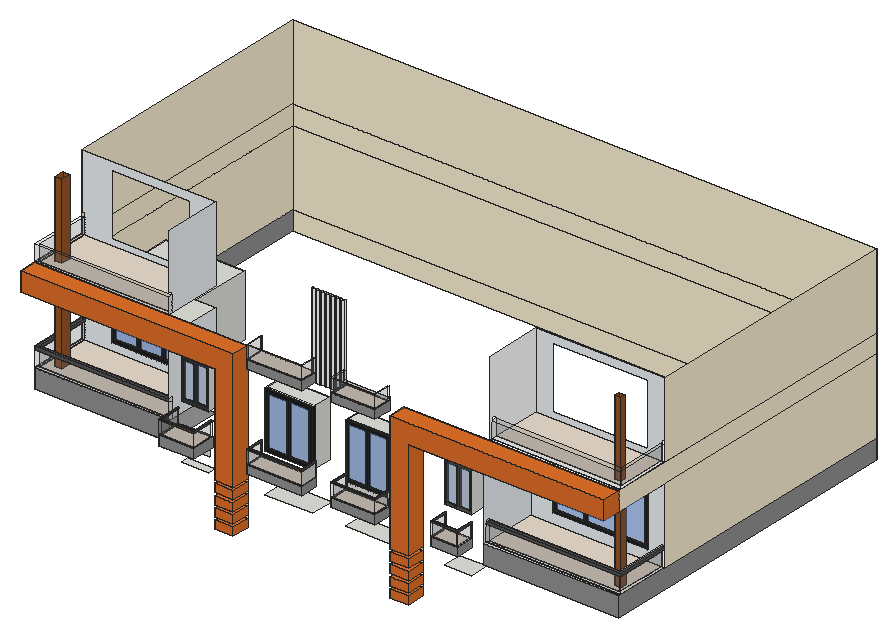
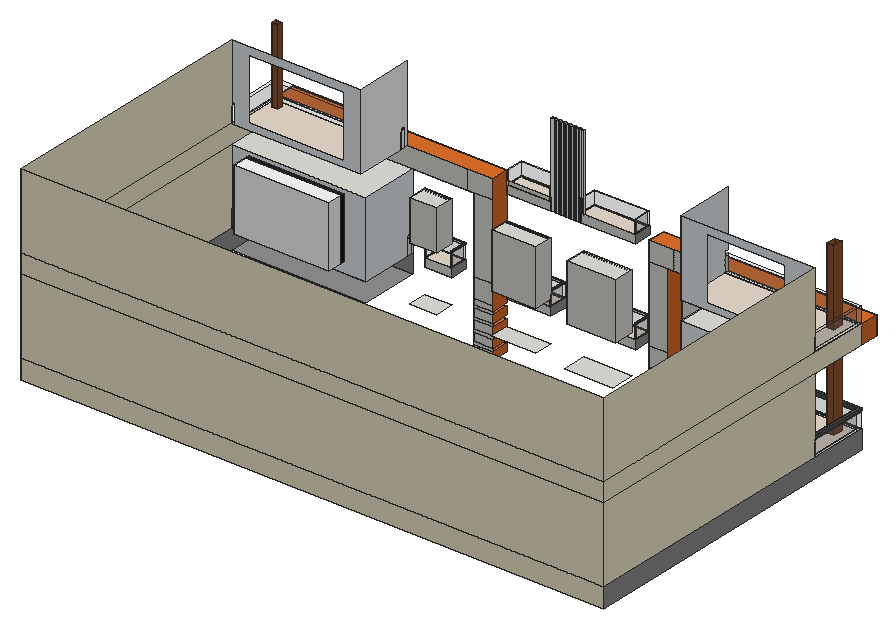
# SketchUp Ruby script. Lengths in inches.
U = 1.inch
M = Sketchup.active_model
def pt(a) = Geom::Point3d.new(a.map { |v| v * U })
def face(e, loops, mat)
  f = e.add_face(loops[0].map { |a| pt(a) })
  loops[1..].each { |l| e.add_face(l.map { |a| pt(a) }).erase! }
  f.material = f.back_material = mat if mat
  f
end
# faces: each face lists its corners as indices into pts; further lists are holes
def faces(e, pts, list, mat = nil) = list.each { |f| face(e, (f[0].is_a?(Array) ? f : [f]).map { |l| l.map { |i| pts[i] } }, mat) }
# xy, xz, yz: faces in a plane at the given z, y or x. An outline is a flat list of corners, or four numbers for a rectangle; further outlines are holes
def ring(l) = l.size == 4 ? [[l[0], l[1]], [l[2], l[1]], [l[2], l[3]], [l[0], l[3]]] : l.each_slice(2).to_a
def flat(e, list, mat, &to3) = list.each { |f| face(e, (f[0].is_a?(Array) ? f : [f]).map { |l| ring(l).map { |u, v| to3.(u, v) } }, mat) }
def xy(e, z, list, mat = nil) = flat(e, list, mat) { |x, y| [x, y, z] }
def xz(e, y, list, mat = nil) = flat(e, list, mat) { |x, z| [x, y, z] }
def yz(e, x, list, mat = nil) = flat(e, list, mat) { |y, z| [x, y, z] }
def lines(e, pts, list) = list.each { |a, b| e.add_line(pt(pts[a]), pt(pts[b])) }
# prism: a flat outline (further loops are holes) pulled along v
def prism(e, loops, v, mat = nil)
  f = face(e, loops, mat); d = Geom::Vector3d.new(v.map { |x| x * U })
  f.pushpull(f.normal.samedirection?(d) ? d.length : -d.length)
end
def box(e, o, s, mat = nil) = prism(e, [[o, [o[0] + s[0], o[1], o[2]], [o[0] + s[0], o[1] + s[1], o[2]], [o[0], o[1] + s[1], o[2]]]], [0, 0, s[2]], mat)
def at(x, y, z, deg = 0) = Geom::Transformation.translation(pt([x, y, z])) * Geom::Transformation.rotation(ORIGIN, Z_AXIS, deg.degrees)
def axes(o, x, y, z) = Geom::Transformation.new([*x, 0, *y, 0, *z, 0, *pt(o).to_a, 1])
def part(name) = M.definitions.add(name)
# library, detail: a bought-in or finely detailed component or shape, given as its bounding box
def library(name, o, s) = part(name).tap { |d| box(d.entities, o, s) }
def detail(e, o, s) = box(e.add_group.entities, o, s)
def put(e, d, t, mat = nil) = e.add_instance(d, t).tap { |i| i.material = mat if mat }
def group(e, t, mat = nil) = e.add_group.tap { |g| g.transformation = t; g.material = mat if mat }.entities
root = M.entities
M.materials.add("Generic").color = [146, 146, 146]
M.materials.add("Generic\#3").color = [226, 112, 41]
M.materials.add("Generic\#4").color = [237, 241, 244]
M.materials.add("Generic\#5").color = [249, 239, 211]
M.materials.add("Generic\#7").color = [232, 220, 205]
M.materials.add("[Color M00]").color = [255, 255, 255]
M.materials.add("[Color M06]").color = [86, 86, 86]
M.materials.add("[Color M07]").color = [58, 58, 58]
M.materials.add("[Color M08]").color = [30, 30, 30]
M.materials.add("[Translucent Glass Blue]").color = [98, 147, 234]
M.materials["[Translucent Glass Blue]"].alpha = 0.27
M.materials.add("[Translucent Glass Blue]1").color = [100, 149, 237]
M.materials["[Translucent Glass Blue]1"].alpha = 0.5
M.materials.add("[Translucent Glass Gray]").color = [119, 119, 119]
M.materials["[Translucent Glass Gray]"].alpha = 0.16
M.materials.add("[Wood Cherry Original]").color = [150, 85, 41]
M.materials.add("[Wood Cherry Original]1").color = [152, 86, 42]
c1 = part("Group\#11")
xy(c1.entities,0,[[0,0,175.8125,6]],"[Color M08]")
xy(c1.entities,7.33,[[7.33,0,56.16,3],[63.49,0,112.32,3],[119.65,0,168.48,3]],"[Color M08]")
xy(c1.entities,131.1,[[7.33,0,56.16,3],[63.49,0,112.32,3],[119.65,0,168.48,3]],"[Color M08]")
xy(c1.entities,138.4375,[[0,0,175.8125,6]],"[Color M08]")
xz(c1.entities,0,[[[0,0,175.8125,0,175.8125,131.1,168.48,131.1,168.48,7.33,119.65,7.33,119.65,131.1,175.8125,131.1,175.8125,138.4375,0,138.4375],[7.33,7.33,56.16,131.1],[63.49,7.33,112.32,131.1]]],"[Color M08]")
xz(c1.entities,3,[[7.33,7.33,56.16,131.1],[63.49,7.33,112.32,131.1],[119.65,7.33,168.48,131.1]],"[Translucent Glass Blue]1")
xz(c1.entities,6,[[0,0,175.8125,138.4375]])
yz(c1.entities,0,[[0,0,6,138.4375]],"[Color M08]")
yz(c1.entities,7.33,[[0,7.33,3,131.1]],"[Color M08]")
yz(c1.entities,56.16,[[0,7.33,3,131.1]],"[Color M08]")
yz(c1.entities,63.49,[[0,7.33,3,131.1]],"[Color M08]")
yz(c1.entities,112.32,[[0,7.33,3,131.1]],"[Color M08]")
yz(c1.entities,119.65,[[0,7.33,3,131.1]],"[Color M08]")
yz(c1.entities,168.48,[[0,7.33,3,131.1]],"[Color M08]")
yz(c1.entities,175.8125,[[0,0,6,138.4375]],"[Color M08]")
c2 = part("Group\#10")
xy(c2.entities,0,[[0,0,98.1875,6]],"[Color M08]")
xy(c2.entities,5.79,[[5.79,0,46.2,3],[51.99,0,92.4,3]],"[Color M08]")
xy(c2.entities,117.02,[[5.79,0,46.2,3],[51.99,0,92.4,3]],"[Color M08]")
xy(c2.entities,122.8125,[[0,0,98.1875,6]],"[Color M08]")
xz(c2.entities,0,[[[0,0,98.1875,122.8125],[5.79,5.79,46.2,117.02],[51.99,5.79,92.4,117.02]]],"[Color M08]")
xz(c2.entities,3,[[5.79,5.79,46.2,117.02],[51.99,5.79,92.4,117.02]],"[Translucent Glass Blue]1")
xz(c2.entities,6,[[0,0,98.1875,122.8125]])
yz(c2.entities,0,[[0,0,6,122.8125]],"[Color M08]")
yz(c2.entities,5.79,[[0,5.79,3,117.02]],"[Color M08]")
yz(c2.entities,46.2,[[0,5.79,3,117.02]],"[Color M08]")
yz(c2.entities,51.99,[[0,5.79,3,117.02]],"[Color M08]")
yz(c2.entities,92.4,[[0,5.79,3,117.02]],"[Color M08]")
yz(c2.entities,98.1875,[[0,0,6,122.8125]],"[Color M08]")
c3 = part("Group\#12")
xy(c3.entities,0,[[0,0,212.5625,7]],"[Color M08]")
xy(c3.entities,6.29,[[6.29,0,68.76,4],[75.05,0,137.52,4],[143.8,0,206.27,4]],"[Color M08]")
xy(c3.entities,131.21,[[6.29,0,68.76,4],[75.05,0,137.52,4],[143.8,0,206.27,4]],"[Color M08]")
xy(c3.entities,137.5,[[0,0,212.5625,7]],"[Color M08]")
xz(c3.entities,0,[[0,0,212.5625,6.29],[0,6.29,6.29,131.21],[68.76,6.29,75.05,131.21],[137.52,6.29,143.8,131.21],[206.27,6.29,212.5625,131.21],
  [0,131.21,212.5625,137.5]],"[Color M08]")
xz(c3.entities,4,[[6.29,6.29,68.76,131.21],[75.05,6.29,137.52,131.21],[143.8,6.29,206.27,131.21]],"[Translucent Glass Blue]1")
xz(c3.entities,7,[[0,0,212.5625,137.5]],"[Color M00]")
yz(c3.entities,0,[[0,0,7,137.5]],"[Color M08]")
yz(c3.entities,6.29,[[0,6.29,4,131.21]],"[Color M08]")
yz(c3.entities,68.76,[[0,6.29,4,131.21]],"[Color M08]")
yz(c3.entities,75.05,[[0,6.29,4,131.21]],"[Color M08]")
yz(c3.entities,137.52,[[0,6.29,4,131.21]],"[Color M08]")
yz(c3.entities,143.8,[[0,6.29,4,131.21]],"[Color M08]")
yz(c3.entities,206.27,[[0,6.29,4,131.21]],"[Color M08]")
yz(c3.entities,212.5625,[[0,0,7,137.5]],"[Color M08]")
c4 = part("Group\#1")
xy(c4.entities,0,[[0,0,60.75,6]],"[Color M07]")
xy(c4.entities,5.51,[[5.51,0,27.62,3],[33.13,0,55.24,3]],"[Color M07]")
xy(c4.entities,84.62,[[5.51,0,27.62,3],[33.13,0,55.24,3]])
xy(c4.entities,90.125,[[0,0,60.75,6]],"[Color M07]")
xz(c4.entities,0,[[[0,0,60.75,90.125],[5.51,5.51,27.62,84.62],[33.13,5.51,55.24,84.62]]],"[Color M07]")
xz(c4.entities,3,[[5.51,5.51,27.62,84.62],[33.13,5.51,55.24,84.62]],"[Translucent Glass Blue]")
xz(c4.entities,6,[[0,0,60.75,90.125]])
yz(c4.entities,0,[[0,0,6,90.125]],"[Color M07]")
yz(c4.entities,5.51,[[0,5.51,3,84.62]],"[Color M07]")
yz(c4.entities,27.62,[[0,5.51,3,84.62]],"[Color M07]")
yz(c4.entities,33.13,[[0,5.51,3,84.62]],"[Color M07]")
yz(c4.entities,55.24,[[0,5.51,3,84.62]],"[Color M07]")
yz(c4.entities,60.75,[[0,0,6,90.125]],"[Color M07]")
c5 = part("Group\#2")
xy(c5.entities,0,[[0,0,60.75,6]],"[Color M06]")
xy(c5.entities,4.875,[[4.875,0,27.9375,3],[32.8125,0,55.875,3]],"[Color M06]")
xy(c5.entities,85.25,[[4.875,0,27.9375,3],[32.8125,0,55.875,3]],"[Color M06]")
xy(c5.entities,90.125,[[0,0,60.75,6]],"[Color M06]")
xz(c5.entities,0,[[[0,0,60.75,90.125],[4.875,4.875,27.9375,85.25],[32.8125,4.875,55.875,85.25]]],"[Color M06]")
xz(c5.entities,3,[[4.875,4.875,27.9375,85.25],[32.8125,4.875,55.875,85.25]],"[Translucent Glass Blue]")
xz(c5.entities,6,[[0,0,60.75,90.125]])
yz(c5.entities,0,[[0,0,6,90.125]],"[Color M06]")
yz(c5.entities,4.875,[[0,4.875,3,85.25]],"[Color M06]")
yz(c5.entities,27.9375,[[0,4.875,3,85.25]],"[Color M06]")
yz(c5.entities,32.8125,[[0,4.875,3,85.25]],"[Color M06]")
yz(c5.entities,55.875,[[0,4.875,3,85.25]],"[Color M06]")
yz(c5.entities,60.75,[[0,0,6,90.125]],"[Color M06]")
xy(root,1321.87,[[643.375,273.75,685.0625,313.625],[1034.5,273.75,1076.1875,313.625]],"Generic\#3")
xy(root,1339.87,[[643.375,273.75,685.0625,313.625],[1034.5,273.75,1076.1875,313.625]],"Generic\#3")
xy(root,1346.37,[[643.375,273.75,685.0625,313.625],[1034.5,273.75,1076.1875,313.625]],"Generic\#3")
xy(root,1364.37,[[643.375,273.75,685.0625,313.625],[1034.5,273.75,1076.1875,313.625]],"Generic\#3")
xy(root,1370.87,[[643.375,273.75,685.0625,313.625],[1034.5,273.75,1076.1875,313.625]],"Generic\#3")
xy(root,1388.87,[[643.375,273.75,685.0625,313.625],[1034.5,273.75,1076.1875,313.625]],"Generic\#3")
xy(root,1395.37,[[643.375,273.75,685.0625,313.625],[1034.5,273.75,1076.1875,313.625]],"Generic\#3")
xy(root,1401.52,[[537.9,313.625,598.65,331.25],[722.84,313.625,830.21,367.6875],[903.71,313.625,1001.9,356.375],[1125.09,313.625,1185.84,356.375]])
xy(root,1411.19,[[1262.61,444.3125,1475.18,486.125]],"[Color M00]")
xy(root,1413.37,[[643.375,273.75,685.0625,313.625],[1034.5,273.75,1076.1875,313.625]],"Generic\#3")
xy(root,1419.87,[[643.375,273.75,685.0625,313.625],[1034.5,273.75,1076.1875,313.625]],"Generic\#3")
xy(root,1424.76,[[276.39,444.3125,452.2,595.9375]])
xy(root,1432.5,[[[209.5,313.625,509.5,444.3125],[234.12,340.02,249.74,361.77]],[[1213,313.625,1513,444.3125],[1483.76,340.63,1497.19,353.98]]],"Generic")
xy(root,1453.875,[[529.46,261.625,607.09,313.625]],"Generic")
xy(root,1456.8125,[[714.9,273.75,838.15,313.625],[903.71,273.75,1001.9,313.625],[1125.09,273.75,1185.84,313.625]],"Generic")
xy(root,1475.25,[[529.46,261.625,529.46,313.625,532.46,313.625,532.46,264.625,604.09,264.625,604.09,313.625,607.09,313.625,607.09,261.625],[714.9,273.75,838.15,276.75],[903.71,273.75,1001.9,276.75],[1125.09,273.75,1185.84,276.75],[714.9,276.75,717.9,313.625],
  [835.15,276.75,838.15,313.625],[903.71,276.75,906.71,313.625],[998.9,276.75,1001.9,313.625],[1125.09,276.75,1128.09,313.625],[1182.84,276.75,1185.84,313.625],
  [209.5,313.625,509.5,320.625],[537.9,313.625,598.65,316.8125],[1213,313.625,1513,319.625],[1213,319.625,1213,327.625,1506,327.625,1506,444.3125,1513,444.3125,1513,319.625],[209.5,320.625,216.5,444.3125],
  [234.12,340.02,249.74,361.77],[1483.76,340.63,1497.19,353.98]])
xy(root,1475.25,[[532.46,264.625,604.09,313.625],[717.9,276.75,835.15,313.625],[906.71,276.75,998.9,313.625],[1128.09,276.75,1182.84,313.625],[[216.5,320.625,509.5,444.3125],[234.12,340.02,249.74,361.77]],
  [[1213,327.625,1506,444.3125],[1483.76,340.63,1497.19,353.98]]],"Generic\#7")
xy(root,1488.02,[[722.84,313.625,830.21,360.5]])
xy(root,1491.07,[[276.39,444.3125,452.2,595.9375]])
xy(root,1491.09,[[903.71,313.625,1001.9,356.375]])
xy(root,1496.57,[[1262.61,444.3125,1475.18,486.125]],"[Color M00]")
xy(root,1505.25,[[529.46,261.625,529.46,313.625,532.46,313.625,532.46,264.625,604.09,264.625,604.09,313.625,607.09,313.625,607.09,261.625],[714.9,273.75,838.15,276.75],[903.71,273.75,1001.9,276.75],[1125.09,273.75,1185.84,276.75],[714.9,276.75,717.9,313.625],
  [835.15,276.75,838.15,313.625],[903.71,276.75,906.71,313.625],[998.9,276.75,1001.9,313.625],[1125.09,276.75,1128.09,313.625],[1182.84,276.75,1185.84,313.625]])
xy(root,1508,[[529.46,261.625,607.09,261.625,607.09,313.625,604.09,313.625,604.09,264.625,532.46,264.625,532.46,313.625,529.46,313.625]],"[Color M06]")
xy(root,1508.25,[[714.9,273.75,838.15,273.75,838.15,313.625,835.15,313.625,835.15,276.75,717.9,276.75,717.9,313.625,714.9,313.625],[903.71,273.75,1001.9,273.75,1001.9,313.625,998.9,313.625,998.9,276.75,906.71,276.75,906.71,313.625,903.71,313.625],[1125.09,273.75,1185.84,273.75,1185.84,313.625,1182.84,313.625,1182.84,276.75,1128.09,276.75,1128.09,313.625,1125.09,313.625]],"[Color M06]")
xy(root,1511.25,[[209.5,313.625,509.5,320.625],[1213,319.625,1213,327.625,1506,327.625,1506,444.3125,1513,444.3125,1513,319.625],[209.5,320.625,216.5,444.3125]])
xy(root,1517.6875,[[1213,319.625,1513,319.625,1513,444.3125,1506,444.3125,1506,327.625,1213,327.625]],"[Color M06]")
xy(root,1518.25,[[209.5,313.625,509.5,313.625,509.5,320.625,216.5,320.625,216.5,444.3125,209.5,444.3125]],"[Color M06]")
xy(root,1523.77,[[537.9,313.625,598.65,331.25],[1125.09,313.625,1185.84,356.375]])
xy(root,1613.9,[[537.9,313.625,598.65,331.25],[722.84,313.625,830.21,360.5],[903.71,313.625,1001.9,356.375],[1125.09,313.625,1185.84,356.375]])
xy(root,1629.51,[[276.39,444.3125,452.2,595.9375]])
xy(root,1634.07,[[1262.61,444.3125,1475.18,486.125]],"[Color M00]")
xy(root,1643.25,[[[209.5,313.625,509.5,444.3125],[234.12,340.02,249.74,361.77]],[[1213,313.625,1513,444.3125],[1483.76,340.63,1497.19,353.98]]])
xy(root,1643.25,[[209.5,273.75,643.375,313.625],[1076.1875,273.75,1513,313.625]],"Generic\#3")
xy(root,1667.5625,[[714.9,273.75,838.15,313.625],[903.71,273.75,1001.9,313.625]],"Generic")
xy(root,1667.5625,[[841.28,310.125,849.21,313.625],[852.34,310.125,860.28,313.625],[863.4,310.125,871.34,313.625],[874.46,310.125,882.4,313.625],[885.53,310.125,893.46,313.625],
  [896.59,310.125,901.53,313.625],[901.53,310.125,903.71,313.625]],"[Color M00]")
xy(root,1686,[[714.9,273.75,838.15,276.75],[903.71,273.75,1001.9,276.75],[714.9,276.75,717.9,313.625],[835.15,276.75,838.15,313.625],[903.71,276.75,906.71,313.625],
  [998.9,276.75,1001.9,313.625],[209.5,313.625,509.5,320.625],[209.5,320.625,216.5,444.3125],[234.12,340.02,249.74,361.77]])
xy(root,1686,[[209.5,273.75,685.0625,313.625],[1034.5,273.75,1513,313.625]],"Generic\#3")
xy(root,1686,[[717.9,276.75,835.15,276.75,835.15,310.125,830.21,310.125,830.21,313.625,717.9,313.625],[906.71,276.75,998.9,313.625],[[216.5,320.625,509.5,444.3125],[234.12,340.02,249.74,361.77]],[[1224.95,333,1506,444.3125],[1480.93,342.75,1494.87,354.3125]]],"Generic\#7")
xy(root,1686,[[830.21,310.125,835.15,313.625],[1224.95,313.625,1513,320.625],[1224.95,320.625,1224.95,333,1506,333,1506,444.3125,1513,444.3125,1513,320.625],[1480.93,342.75,1494.87,354.3125]],"[Color M00]")
xz(root,261.625,[[529.46,1453.875,607.09,1475.25]],"Generic")
xz(root,261.625,[[529.46,1505.25,607.09,1508]],"[Color M06]")
xz(root,261.625,[[529.46,1475.25,607.09,1505.25]],"[Translucent Glass Gray]")
xz(root,264.625,[[532.46,1505.25,604.09,1508]])
xz(root,264.625,[[532.46,1475.25,604.09,1505.25]],"[Translucent Glass Gray]")
xz(root,273.75,[[714.9,1456.8125,838.15,1475.25],[903.71,1456.8125,1001.9,1475.25],[1125.09,1456.8125,1185.84,1475.25],[714.9,1667.5625,838.15,1686],[903.71,1667.5625,1001.9,1686]],"Generic")
xz(root,273.75,[[643.375,1321.87,685.0625,1339.87],[1034.5,1321.87,1076.1875,1339.87],[643.375,1346.37,685.0625,1364.37],[1034.5,1346.37,1076.1875,1364.37],[643.375,1370.87,685.0625,1388.87],
  [1034.5,1370.87,1076.1875,1388.87],[643.375,1395.37,685.0625,1413.37],[1034.5,1395.37,1076.1875,1413.37],[643.375,1419.87,685.0625,1419.87,685.0625,1686,209.5,1686,209.5,1643.25,643.375,1643.25],[1034.5,1419.87,1076.1875,1419.87,1076.1875,1643.25,1513,1643.25,1513,1686,1034.5,1686]],"Generic\#3")
xz(root,273.75,[[714.9,1505.25,838.15,1508.25],[903.71,1505.25,1001.9,1508.25],[1125.09,1505.25,1185.84,1508.25]],"[Color M06]")
xz(root,273.75,[[714.9,1475.25,838.15,1505.25],[903.71,1475.25,1001.9,1505.25],[1125.09,1475.25,1185.84,1505.25],[714.9,1686,838.15,1716],[903.71,1686,1001.9,1716]],"[Translucent Glass Gray]")
xz(root,276.75,[[717.9,1505.25,835.15,1508.25],[906.71,1505.25,998.9,1508.25],[1128.09,1505.25,1182.84,1508.25]])
xz(root,276.75,[[717.9,1475.25,835.15,1505.25],[906.71,1475.25,998.9,1505.25],[1128.09,1475.25,1182.84,1505.25],[717.9,1686,835.15,1716],[906.71,1686,998.9,1716]],"[Translucent Glass Gray]")
xz(root,310.125,[[841.28,1667.5625,849.21,1854],[852.34,1667.5625,860.28,1854],[863.4,1667.5625,871.34,1854],[874.46,1667.5625,882.4,1854],[885.53,1667.5625,893.46,1854],
  [896.59,1667.5625,903.71,1854],[830.21,1686,835.15,1686,835.15,1719,838.15,1719,838.15,1854,830.21,1854]],"[Color M00]")
xz(root,313.625,[[643.375,1321.87,685.0625,1339.87],[1034.5,1321.87,1076.1875,1339.87],[643.375,1339.87,685.0625,1346.37],[1034.5,1339.87,1076.1875,1346.37],[643.375,1346.37,685.0625,1364.37],
  [1034.5,1346.37,1076.1875,1364.37],[643.375,1364.37,685.0625,1370.87],[1034.5,1364.37,1076.1875,1370.87],[643.375,1370.87,685.0625,1388.87],[1034.5,1370.87,1076.1875,1388.87],
  [643.375,1388.87,685.0625,1395.37],[1034.5,1388.87,1076.1875,1395.37],[643.375,1395.37,685.0625,1413.37],[1034.5,1395.37,1076.1875,1413.37],[643.375,1413.37,685.0625,1419.87],
  [1034.5,1413.37,1076.1875,1419.87],[643.375,1419.87,685.0625,1432.5],[1034.5,1419.87,1076.1875,1432.5],[643.375,1432.5,685.0625,1475.25],[1034.5,1432.5,1076.1875,1475.25],
  [529.46,1453.875,607.09,1475.25],[714.9,1456.8125,838.15,1475.25],[903.71,1456.8125,1001.9,1475.25],[1125.09,1456.8125,1185.84,1475.25],[643.375,1475.25,685.0625,1643.25],
  [714.9,1475.25,717.9,1505.25],[835.15,1475.25,838.15,1505.25],[903.71,1475.25,906.71,1491.09],[906.71,1475.25,998.9,1491.09],[998.9,1475.25,1001.9,1491.09],
  [1034.5,1475.25,1076.1875,1643.25],[1125.09,1475.25,1128.09,1505.25],[1182.84,1475.25,1185.84,1505.25],[903.71,1491.09,906.71,1505.25],[998.9,1491.09,1001.9,1505.25],
  [714.9,1505.25,717.9,1508.25],[835.15,1505.25,838.15,1508.25],[903.71,1505.25,906.71,1508.25],[998.9,1505.25,1001.9,1508.25],[1125.09,1505.25,1128.09,1508.25],
  [1182.84,1505.25,1185.84,1508.25],[209.5,1643.25,629.5,1686],[629.5,1643.25,685.0625,1686],[1034.5,1643.25,1093,1686],[1093,1643.25,1513,1686],
  [714.9,1667.5625,838.15,1686],[903.71,1667.5625,1001.9,1686],[714.9,1686,717.9,1716],[835.15,1686,838.15,1716],[903.71,1686,906.71,1693.92],
  [906.71,1686,998.9,1693.92],[998.9,1686,1001.9,1693.92]])
xz(root,313.625,[[209.5,1432.5,509.5,1475.25],[1213,1432.5,1513,1475.25]],"Generic")
xz(root,313.625,[[838.15,1667.5625,841.28,1854],[841.28,1667.5625,849.21,1854],[849.21,1667.5625,852.34,1854],[852.34,1667.5625,860.28,1854],[860.28,1667.5625,863.4,1854],
  [863.4,1667.5625,871.34,1854],[871.34,1667.5625,874.46,1854],[874.46,1667.5625,882.4,1854],[882.4,1667.5625,885.53,1854],[885.53,1667.5625,893.46,1854],
  [893.46,1667.5625,896.59,1854],[896.59,1667.5625,903.71,1854],[830.21,1686,830.21,1854,838.15,1854,838.15,1719,835.15,1719,835.15,1686]],"[Color M00]")
xz(root,313.625,[[209.5,1511.25,509.5,1518.25]],"[Color M06]")
xz(root,313.625,[[209.5,1475.25,509.5,1511.25],[209.5,1686,509.5,1722]],"[Translucent Glass Gray]")
xz(root,316.8125,[[537.9,1432.5,598.65,1475.25]])
xz(root,319.625,[[1213,1511.25,1513,1517.6875]],"[Color M06]")
xz(root,319.625,[[1213,1475.25,1513,1511.25]],"[Translucent Glass Gray]")
xz(root,320.625,[[216.5,1511.25,509.5,1518.25]],"[Color M06]")
xz(root,320.625,[[216.5,1475.25,509.5,1511.25],[216.5,1686,509.5,1722],[1224.95,1686,1513,1722]],"[Translucent Glass Gray]")
xz(root,327.625,[[1213,1511.25,1506,1517.6875]],"[Color M06]")
xz(root,327.625,[[1213,1475.25,1506,1511.25]],"[Translucent Glass Gray]")
xz(root,331.25,[[537.9,1523.77,598.65,1613.9]])
xz(root,333,[[1224.95,1686,1506,1722]],"[Translucent Glass Gray]")
xz(root,340.02,[[234.12,1475.25,249.74,1643.25],[234.12,1686,249.74,1854]],"[Wood Cherry Original]1")
xz(root,340.63,[[1483.76,1475.25,1497.19,1643.25]],"[Wood Cherry Original]")
xz(root,342.75,[[1480.93,1686,1494.87,1854]],"[Wood Cherry Original]")
xz(root,353.98,[[1483.76,1475.25,1497.19,1643.25]],"[Wood Cherry Original]")
xz(root,354.3125,[[1480.93,1686,1494.87,1854]],"[Wood Cherry Original]")
xz(root,356.375,[[903.71,1491.09,1001.9,1613.9],[1125.09,1523.77,1185.84,1613.9]])
xz(root,360.5,[[722.84,1488.02,830.21,1613.9]])
xz(root,361.77,[[234.12,1475.25,249.74,1643.25],[234.12,1686,249.74,1854]],"[Wood Cherry Original]1")
xz(root,444.3125,[[209.5,1475.25,216.5,1511.25],[209.5,1511.25,216.5,1518.25],[209.5,1686,216.5,1722]])
xz(root,444.3125,[[[216.5,1475.25,509.5,1475.25,509.5,1643.25,209.5,1643.25,209.5,1518.25,216.5,1518.25],[276.39,1491.07,452.2,1629.51]],[[1213,1475.25,1506,1475.25,1506,1517.6875,1513,1517.6875,1513,1643.25,1213,1643.25],[1262.61,1496.57,1475.18,1634.07]],[[216.5,1686,509.5,1686,509.5,1854,209.5,1854,209.5,1729,216.5,1729],[276.39,1698.82,452.2,1837.26]],[[1224.95,1686,1506,1686,1506,1728.4375,1513,1728.4375,1513,1854,1224.95,1854],[1262.61,1699.69,1475.18,1837.19]]],"Generic\#4")
xz(root,486.125,[[1262.61,1496.57,1475.18,1634.07]],"[Color M00]")
xz(root,595.9375,[[276.39,1491.07,452.2,1629.51]])
xz(root,1033.625,[[209.5,1432.5,1513,1475.25],[209.5,1475.25,1513,1643.25],[209.5,1643.25,1513,1686],[209.5,1686,1513,1854]],"Generic\#5")
yz(root,209.5,[[313.625,1432.5,1033.625,1475.25]],"Generic")
yz(root,209.5,[[273.75,1643.25,313.625,1686]],"Generic\#3")
yz(root,209.5,[[444.3125,1475.25,1033.625,1643.25],[313.625,1643.25,1033.625,1686],[444.3125,1686,1033.625,1854]],"Generic\#5")
yz(root,209.5,[[313.625,1511.25,444.3125,1518.25]],"[Color M06]")
yz(root,209.5,[[313.625,1475.25,444.3125,1511.25],[313.625,1686,444.3125,1722]],"[Translucent Glass Gray]")
yz(root,216.5,[[320.625,1511.25,444.3125,1518.25]],"[Color M06]")
yz(root,216.5,[[320.625,1475.25,444.3125,1511.25],[320.625,1686,444.3125,1722]],"[Translucent Glass Gray]")
yz(root,234.12,[[340.02,1475.25,361.77,1643.25],[340.02,1686,361.77,1854]],"[Wood Cherry Original]1")
yz(root,249.74,[[340.02,1475.25,361.77,1643.25],[340.02,1686,361.77,1854]],"[Wood Cherry Original]1")
yz(root,276.39,[[444.3125,1491.07,595.9375,1629.51]])
yz(root,452.2,[[444.3125,1491.07,595.9375,1629.51]])
yz(root,509.5,[[313.625,1475.25,320.625,1511.25],[313.625,1511.25,320.625,1518.25],[313.625,1686,320.625,1722]])
yz(root,509.5,[[320.625,1475.25,320.625,1518.25,313.625,1518.25,313.625,1643.25,444.3125,1643.25,444.3125,1475.25],[320.625,1686,320.625,1729,313.625,1729,313.625,1854,444.3125,1854,444.3125,1686]],"Generic\#4")
yz(root,529.46,[[261.625,1453.875,313.625,1475.25]],"Generic")
yz(root,529.46,[[261.625,1505.25,313.625,1508]],"[Color M06]")
yz(root,529.46,[[261.625,1475.25,313.625,1505.25]],"[Translucent Glass Gray]")
yz(root,532.46,[[264.625,1505.25,313.625,1508]],"[Color M06]")
yz(root,532.46,[[264.625,1475.25,313.625,1505.25]],"[Translucent Glass Gray]")
yz(root,537.9,[[313.625,1523.77,331.25,1613.9]])
yz(root,598.65,[[313.625,1523.77,331.25,1613.9]])
yz(root,604.09,[[264.625,1505.25,313.625,1508]],"[Color M06]")
yz(root,604.09,[[264.625,1475.25,313.625,1505.25]],"[Translucent Glass Gray]")
yz(root,607.09,[[261.625,1453.875,313.625,1475.25]],"Generic")
yz(root,607.09,[[261.625,1505.25,313.625,1508]],"[Color M06]")
yz(root,607.09,[[261.625,1475.25,313.625,1505.25]],"[Translucent Glass Gray]")
yz(root,643.375,[[273.75,1321.87,313.625,1339.87],[273.75,1346.37,313.625,1364.37],[273.75,1370.87,313.625,1388.87],[273.75,1395.37,313.625,1413.37],[273.75,1419.87,313.625,1643.25]],"Generic\#3")
yz(root,685.0625,[[273.75,1321.87,313.625,1339.87],[273.75,1346.37,313.625,1364.37],[273.75,1370.87,313.625,1388.87],[273.75,1395.37,313.625,1413.37],[273.75,1419.87,313.625,1686]],"Generic\#3")
yz(root,714.9,[[273.75,1456.8125,313.625,1475.25],[273.75,1667.5625,313.625,1686]],"Generic")
yz(root,714.9,[[273.75,1505.25,313.625,1508.25]],"[Color M06]")
yz(root,714.9,[[273.75,1475.25,313.625,1505.25],[273.75,1686,313.625,1716]],"[Translucent Glass Gray]")
yz(root,717.9,[[276.75,1505.25,313.625,1508.25]],"[Color M06]")
yz(root,717.9,[[276.75,1475.25,313.625,1505.25],[276.75,1686,313.625,1716]],"[Translucent Glass Gray]")
yz(root,722.84,[[313.625,1488.02,360.5,1613.9]])
yz(root,830.21,[[313.625,1488.02,360.5,1613.9]])
yz(root,830.21,[[310.125,1686,313.625,1854]],"[Color M00]")
yz(root,835.15,[[276.75,1475.25,313.625,1505.25]])
yz(root,835.15,[[310.125,1686,313.625,1716]],"[Color M00]")
yz(root,835.15,[[276.75,1505.25,313.625,1508.25]],"[Color M06]")
yz(root,835.15,[[276.75,1686,310.125,1716]],"[Translucent Glass Gray]")
yz(root,838.15,[[273.75,1456.8125,313.625,1475.25],[273.75,1667.5625,313.625,1686]],"Generic")
yz(root,838.15,[[273.75,1505.25,313.625,1508.25]],"[Color M06]")
yz(root,838.15,[[273.75,1475.25,313.625,1505.25],[273.75,1686,313.625,1716]],"[Translucent Glass Gray]")
yz(root,841.28,[[310.125,1667.5625,313.625,1854]],"[Color M00]")
yz(root,849.21,[[310.125,1667.5625,313.625,1854]],"[Color M00]")
yz(root,852.34,[[310.125,1667.5625,313.625,1854]],"[Color M00]")
yz(root,860.28,[[310.125,1667.5625,313.625,1854]],"[Color M00]")
yz(root,863.4,[[310.125,1667.5625,313.625,1854]],"[Color M00]")
yz(root,871.34,[[310.125,1667.5625,313.625,1854]],"[Color M00]")
yz(root,874.46,[[310.125,1667.5625,313.625,1854]],"[Color M00]")
yz(root,882.4,[[310.125,1667.5625,313.625,1854]],"[Color M00]")
yz(root,885.53,[[310.125,1667.5625,313.625,1854]],"[Color M00]")
yz(root,893.46,[[310.125,1667.5625,313.625,1854]],"[Color M00]")
yz(root,896.59,[[310.125,1667.5625,313.625,1854]],"[Color M00]")
yz(root,903.71,[[313.625,1491.09,356.375,1613.9]])
yz(root,903.71,[[273.75,1456.8125,313.625,1475.25],[273.75,1667.5625,310.125,1686]],"Generic")
yz(root,903.71,[[310.125,1667.5625,313.625,1686],[310.125,1686,313.625,1693.92]],"[Color M00]")
yz(root,903.71,[[273.75,1505.25,313.625,1508.25]],"[Color M06]")
yz(root,903.71,[[273.75,1475.25,313.625,1505.25],[273.75,1686,310.125,1716]],"[Translucent Glass Gray]")
yz(root,906.71,[[276.75,1505.25,313.625,1508.25]],"[Color M06]")
yz(root,906.71,[[276.75,1475.25,313.625,1505.25],[276.75,1686,313.625,1716]],"[Translucent Glass Gray]")
yz(root,998.9,[[276.75,1505.25,313.625,1508.25]],"[Color M06]")
yz(root,998.9,[[276.75,1475.25,313.625,1505.25],[276.75,1686,313.625,1716]],"[Translucent Glass Gray]")
yz(root,1001.9,[[313.625,1491.09,356.375,1613.9]])
yz(root,1001.9,[[273.75,1456.8125,313.625,1475.25],[273.75,1667.5625,313.625,1686]],"Generic")
yz(root,1001.9,[[273.75,1505.25,313.625,1508.25]],"[Color M06]")
yz(root,1001.9,[[273.75,1475.25,313.625,1505.25],[273.75,1686,313.625,1716]],"[Translucent Glass Gray]")
yz(root,1034.5,[[273.75,1321.87,313.625,1339.87],[273.75,1346.37,313.625,1364.37],[273.75,1370.87,313.625,1388.87],[273.75,1395.37,313.625,1413.37],[273.75,1419.87,313.625,1686]],"Generic\#3")
yz(root,1076.1875,[[273.75,1321.87,313.625,1339.87],[273.75,1346.37,313.625,1364.37],[273.75,1370.87,313.625,1388.87],[273.75,1395.37,313.625,1413.37],[273.75,1419.87,313.625,1643.25]],"Generic\#3")
yz(root,1125.09,[[313.625,1523.77,356.375,1613.9]])
yz(root,1125.09,[[273.75,1456.8125,313.625,1475.25]],"Generic")
yz(root,1125.09,[[273.75,1505.25,313.625,1508.25]],"[Color M06]")
yz(root,1125.09,[[273.75,1475.25,313.625,1505.25]],"[Translucent Glass Gray]")
yz(root,1128.09,[[276.75,1505.25,313.625,1508.25]],"[Color M06]")
yz(root,1128.09,[[276.75,1475.25,313.625,1505.25]],"[Translucent Glass Gray]")
yz(root,1182.84,[[276.75,1505.25,313.625,1508.25]],"[Color M06]")
yz(root,1182.84,[[276.75,1475.25,313.625,1505.25]],"[Translucent Glass Gray]")
yz(root,1185.84,[[313.625,1523.77,356.375,1613.9]])
yz(root,1185.84,[[273.75,1456.8125,313.625,1475.25]],"Generic")
yz(root,1185.84,[[273.75,1505.25,313.625,1508.25]],"[Color M06]")
yz(root,1185.84,[[273.75,1475.25,313.625,1505.25]],"[Translucent Glass Gray]")
yz(root,1213,[[319.625,1475.25,327.625,1511.25],[319.625,1511.25,327.625,1517.6875]])
yz(root,1213,[[313.625,1475.25,319.625,1475.25,319.625,1517.6875,327.625,1517.6875,327.625,1475.25,444.3125,1475.25,444.3125,1643.25,313.625,1643.25]],"Generic\#4")
yz(root,1224.95,[[313.625,1686,320.625,1686,320.625,1728.4375,333,1728.4375,333,1686,444.3125,1686,444.3125,1854,313.625,1854],[320.625,1686,333,1722]],"[Color M00]")
yz(root,1262.61,[[444.3125,1496.57,486.125,1634.07]],"[Color M00]")
yz(root,1475.18,[[444.3125,1496.57,486.125,1634.07]],"[Color M00]")
yz(root,1480.93,[[342.75,1686,354.3125,1854]],"[Wood Cherry Original]")
yz(root,1483.76,[[340.63,1475.25,353.98,1643.25]],"[Wood Cherry Original]")
yz(root,1494.87,[[342.75,1686,354.3125,1854]],"[Wood Cherry Original]")
yz(root,1497.19,[[340.63,1475.25,353.98,1643.25]],"[Wood Cherry Original]")
yz(root,1506,[[327.625,1511.25,444.3125,1517.6875]])
yz(root,1506,[[327.625,1475.25,444.3125,1511.25],[333,1686,444.3125,1722]],"[Translucent Glass Gray]")
yz(root,1513,[[313.625,1432.5,1033.625,1475.25]],"Generic")
yz(root,1513,[[273.75,1643.25,313.625,1686]],"Generic\#3")
yz(root,1513,[[444.3125,1475.25,1033.625,1643.25],[313.625,1643.25,1033.625,1686],[444.3125,1686,1033.625,1854]],"Generic\#5")
yz(root,1513,[[319.625,1511.25,444.3125,1517.6875]],"[Color M06]")
yz(root,1513,[[319.625,1475.25,444.3125,1511.25],[320.625,1686,444.3125,1722]],"[Translucent Glass Gray]")
p = [[598.65,313.625,1432.5],[598.65,316.8125,1432.5],[537.9,313.625,1432.5],[537.9,316.8125,1432.5]]
lines(root,p,[[0,1],[2,3]])
g1 = group(root,at(722.84,313.625,1488.02))
xy(g1,0,[[0,0,107.375,6]],"[Color M08]")
xy(g1,7.58,[[7.58,0,49.9,3],[57.48,0,99.79,3]],"[Color M08]")
xy(g1,118.29,[[7.58,0,49.9,3],[57.48,0,99.79,3]],"[Color M08]")
xy(g1,125.875,[[0,0,107.375,6]],"[Color M08]")
xz(g1,0,[[[0,0,107.375,125.875],[7.58,7.58,49.9,118.29],[57.48,7.58,99.79,118.29]]],"[Color M08]")
xz(g1,3,[[7.58,7.58,49.9,118.29],[57.48,7.58,99.79,118.29]],"[Translucent Glass Blue]1")
xz(g1,6,[[0,0,107.375,125.875]])
yz(g1,0,[[0,0,6,125.875]],"[Color M08]")
yz(g1,7.58,[[0,7.58,3,118.29]],"[Color M08]")
yz(g1,49.9,[[0,7.58,3,118.29]],"[Color M08]")
yz(g1,57.48,[[0,7.58,3,118.29]],"[Color M08]")
yz(g1,99.79,[[0,7.58,3,118.29]],"[Color M08]")
yz(g1,107.375,[[0,0,6,125.875]],"[Color M08]")
put(root,c1,at(276.39,444.3125,1491.07))
put(root,c2,at(903.71,313.625,1491.09))
put(root,c3,at(1262.11,444.625,1496.57))
put(root,c4,at(537.9,313.625,1523.77))
put(root,c5,at(1125.09,313.625,1523.77))
